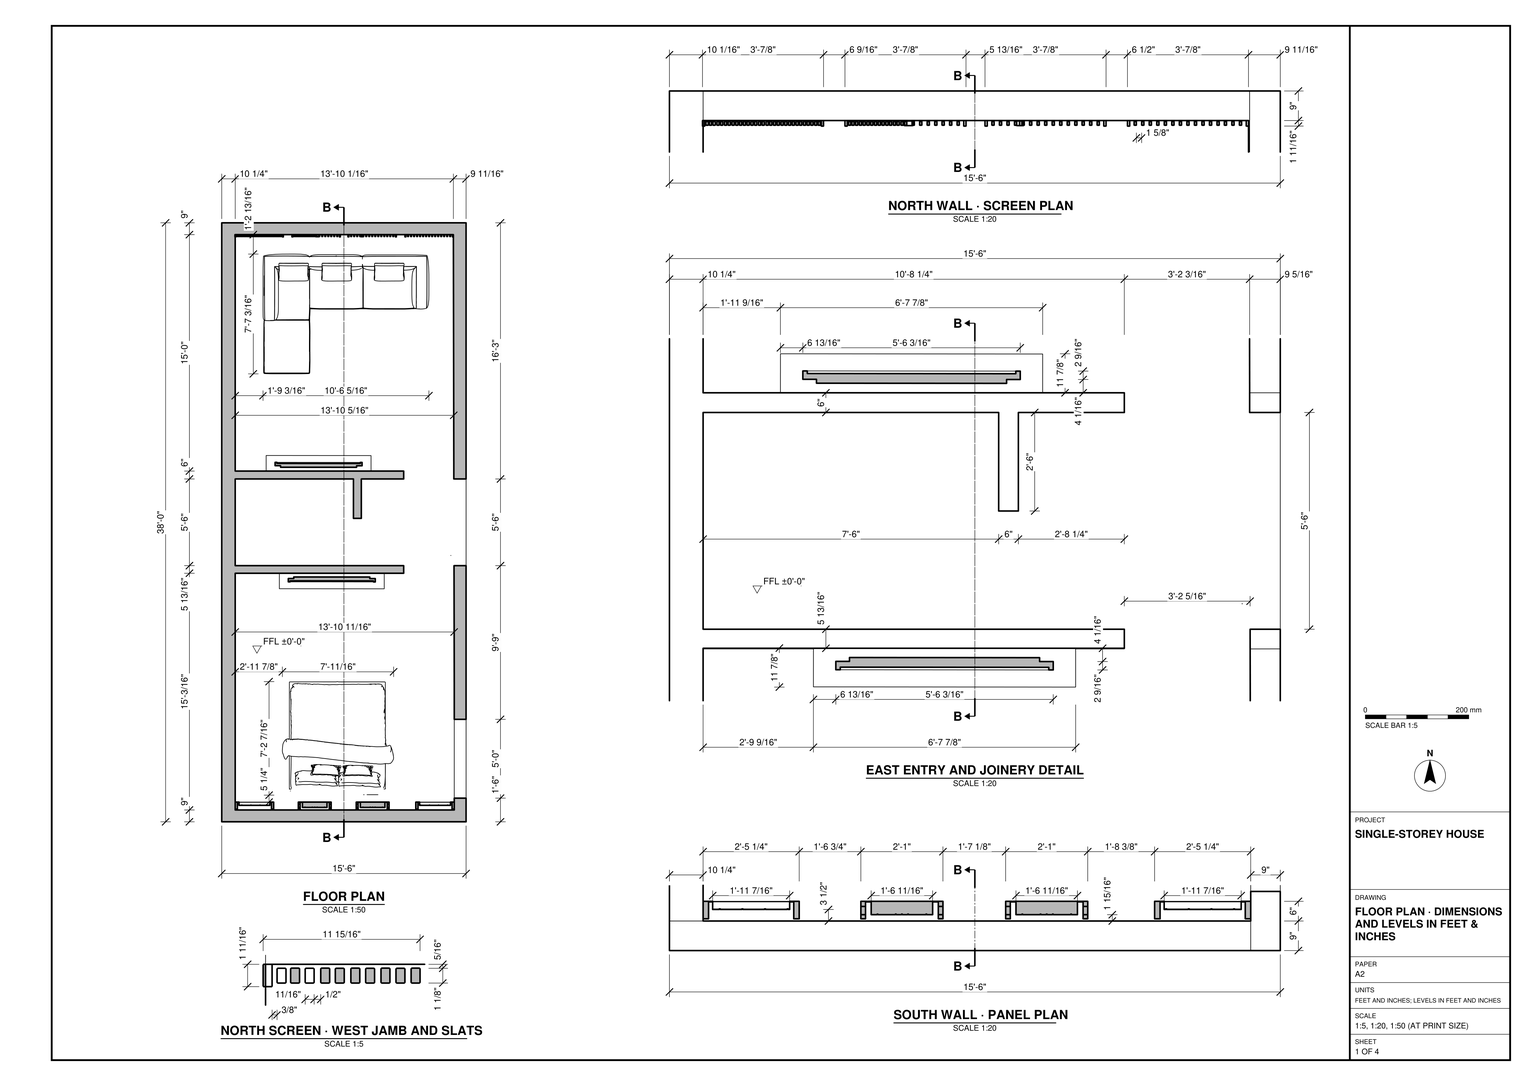
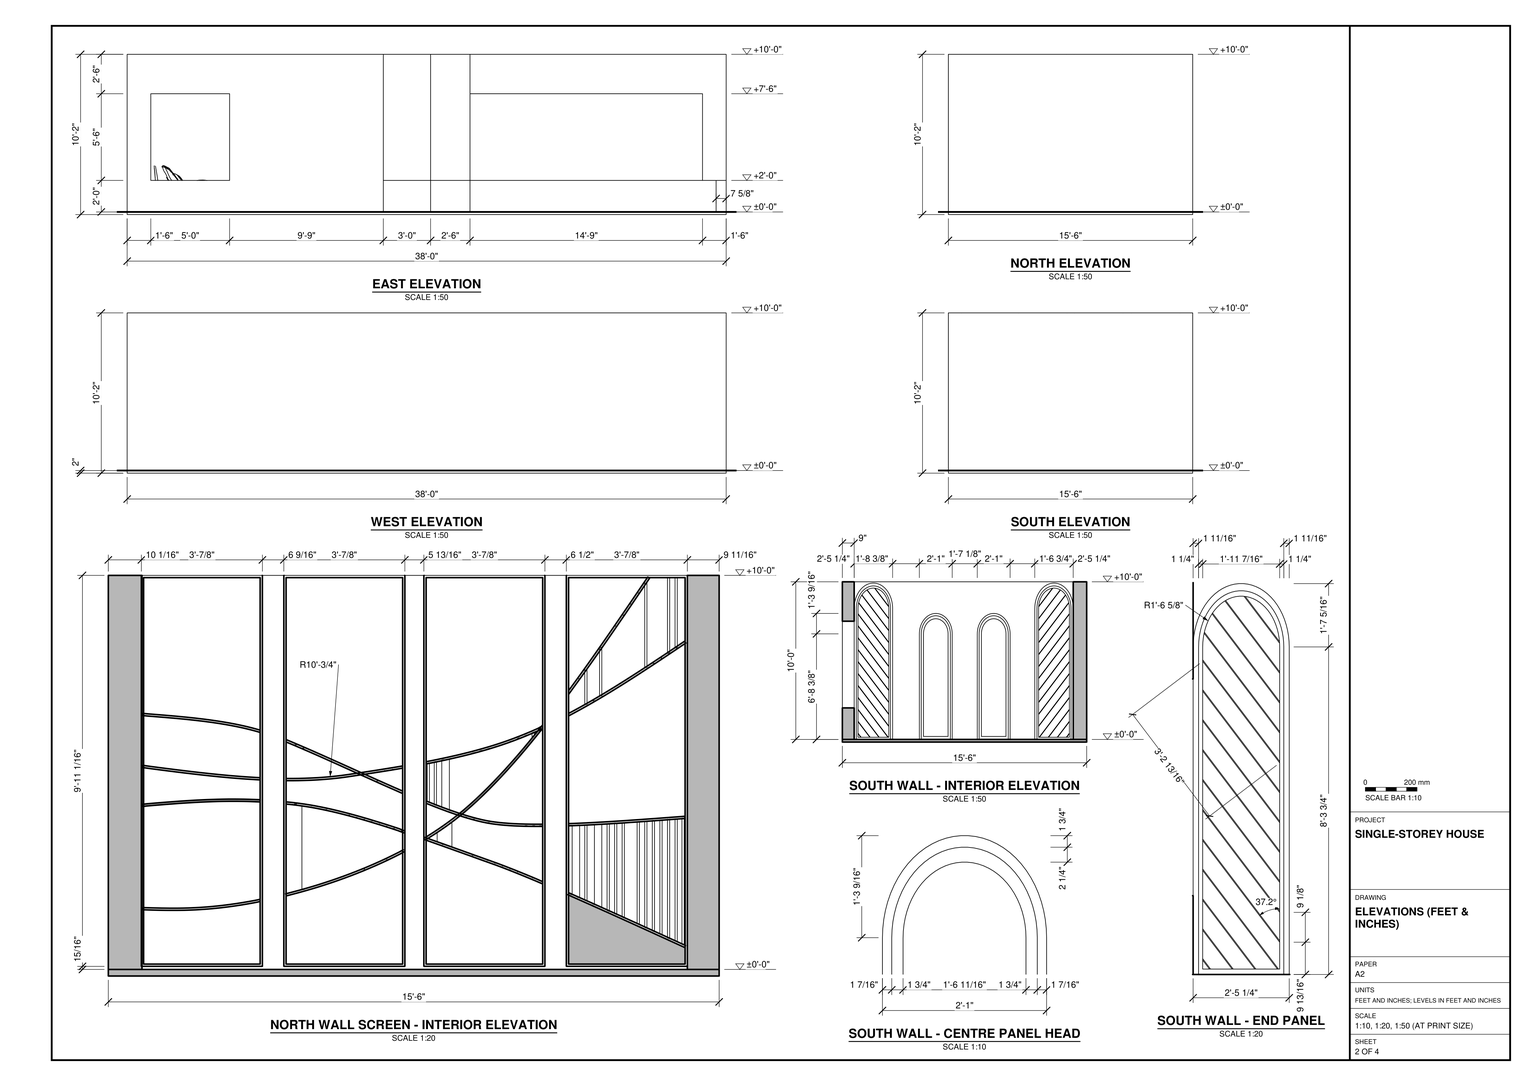
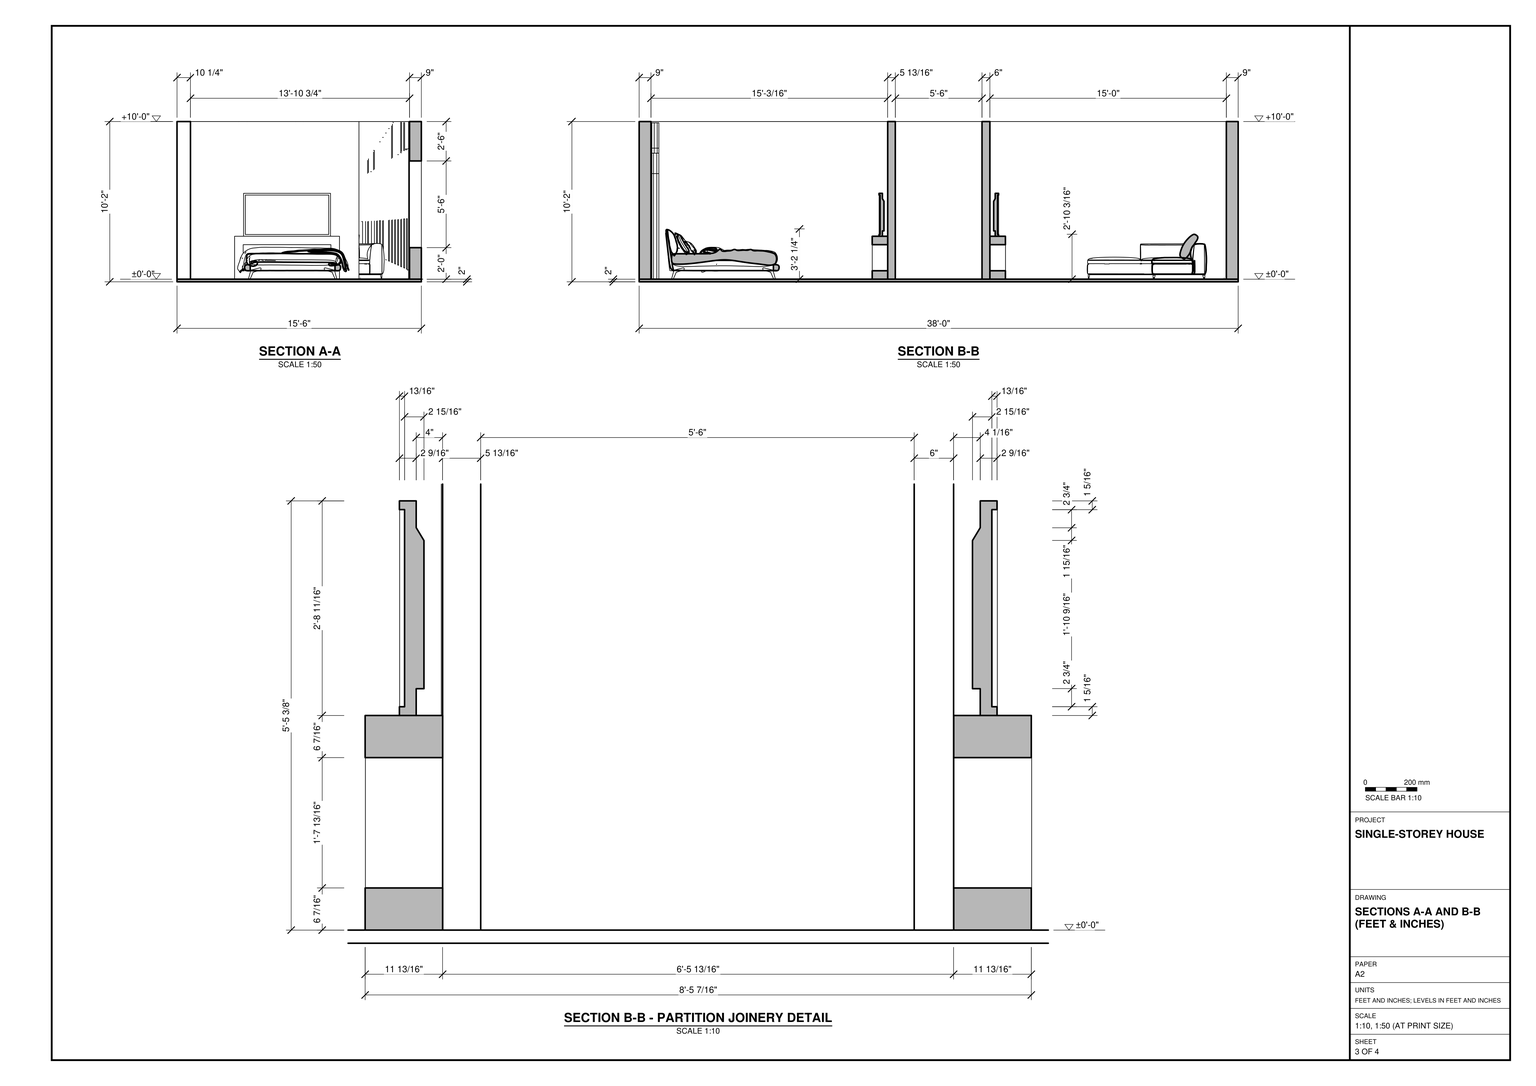
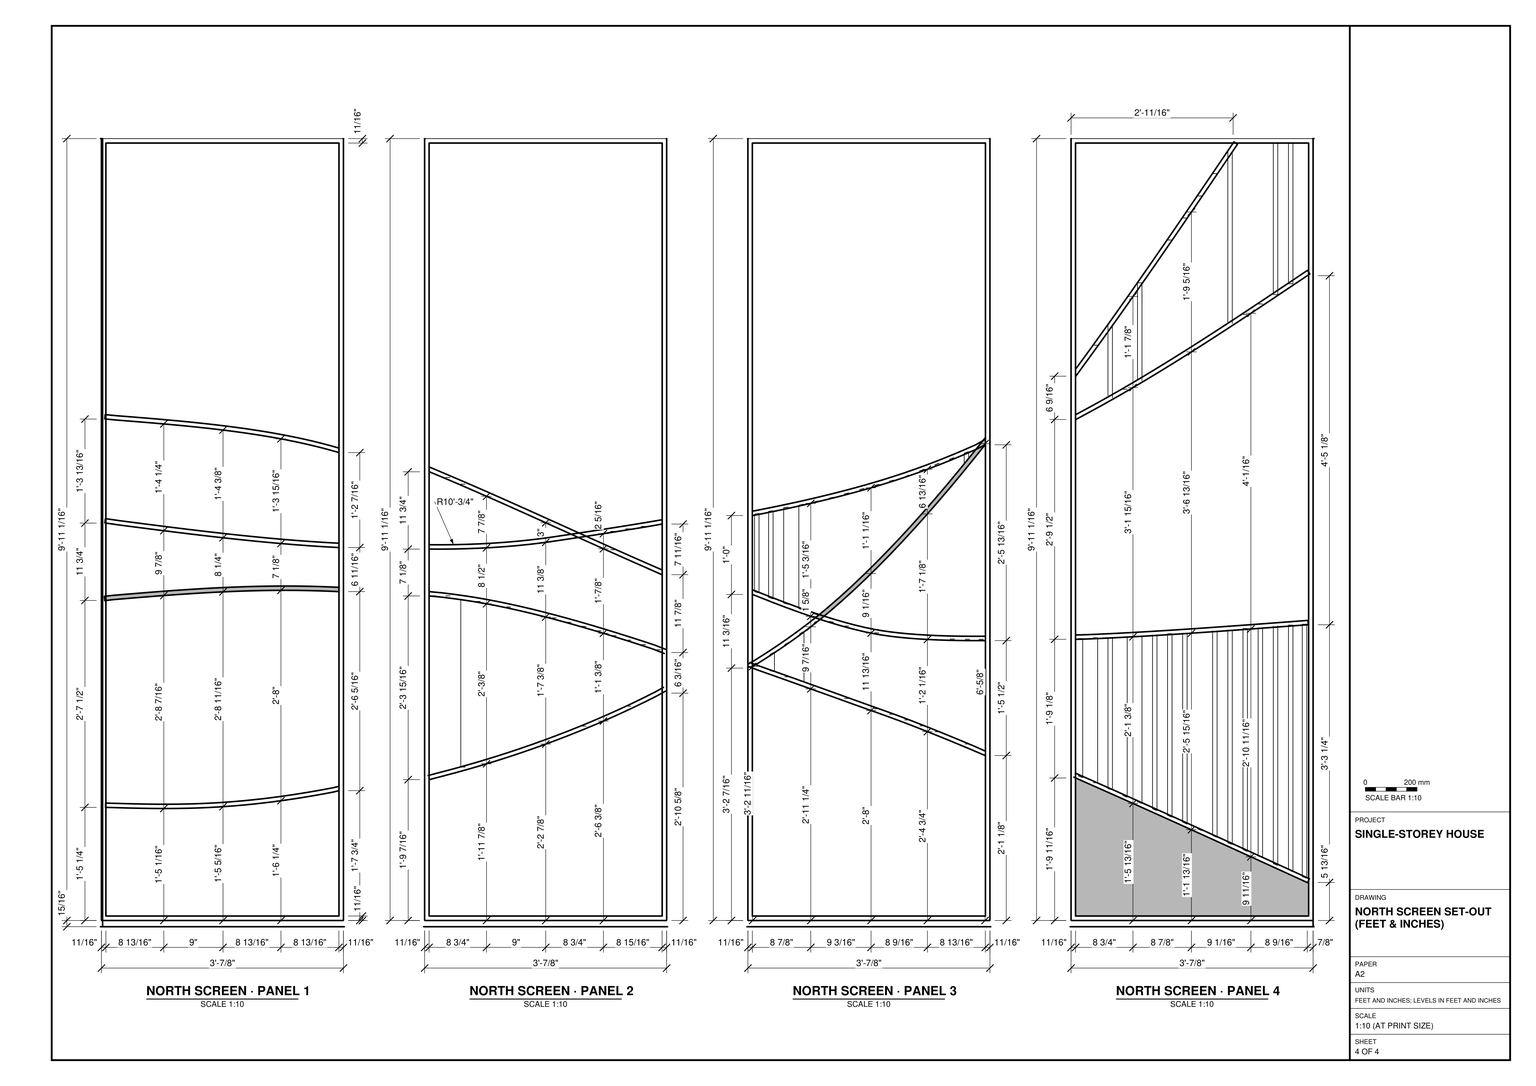
Build the house in SketchUp from task_files/diagram_01.pdf. Work in feet and inches. The rectangular footprint is 15'-6" east to west by 38'-0" north to south. Set the finished floor at ±0'-0". The overall height is 10'-2", measured from the underside of the floor slab to the wall tops.

Model the slab and perimeter walls with the thicknesses shown in plan and section. Keep the west wall continuous. Form the central entry and the two room openings in the east wall, matching their positions, sills and heads to the east elevation. Build the transverse partitions on either side of the entry, including the short return on the northern partition. Fit the low media units and their upright screens against the partition faces that look into the rooms.

Place the sectional sofa at the north end, with its chaise on the west. Behind it, model the framed screen with curved rails and vertical slats. Place the bed with its head toward the south wall and model the arched wall panels behind it, distinguishing the taller end panels from the shorter centre pair. Use the plan for furniture footprints and the interior elevations for joinery profiles. Decor and loose items may be any suitable library components. Keep shell elements and individual furniture and joinery pieces in separate groups or components, and use components for repeated parts. Save one SketchUp model as output_files/single_storey_house_with_screens_and_partition_joinery.skp.

# SketchUp Ruby script. Lengths in inches.
U = 1.inch
M = Sketchup.active_model
def pt(a) = Geom::Point3d.new(a.map { |v| v * U })
def face(e, loops, mat)
  f = e.add_face(loops[0].map { |a| pt(a) })
  loops[1..].each { |l| e.add_face(l.map { |a| pt(a) }).erase! }
  f.material = f.back_material = mat if mat
  f
end
# faces: each face lists its corners as indices into pts; further lists are holes
def faces(e, pts, list, mat = nil) = list.each { |f| face(e, (f[0].is_a?(Array) ? f : [f]).map { |l| l.map { |i| pts[i] } }, mat) }
# xy, xz, yz: faces in a plane at the given z, y or x. An outline is a flat list of corners, or four numbers for a rectangle; further outlines are holes
def ring(l) = l.size == 4 ? [[l[0], l[1]], [l[2], l[1]], [l[2], l[3]], [l[0], l[3]]] : l.each_slice(2).to_a
def flat(e, list, mat, &to3) = list.each { |f| face(e, (f[0].is_a?(Array) ? f : [f]).map { |l| ring(l).map { |u, v| to3.(u, v) } }, mat) }
def xy(e, z, list, mat = nil) = flat(e, list, mat) { |x, y| [x, y, z] }
def xz(e, y, list, mat = nil) = flat(e, list, mat) { |x, z| [x, y, z] }
def yz(e, x, list, mat = nil) = flat(e, list, mat) { |y, z| [x, y, z] }
def lines(e, pts, list) = list.each { |a, b| e.add_line(pt(pts[a]), pt(pts[b])) }
# prism: a flat outline (further loops are holes) pulled along v
def prism(e, loops, v, mat = nil)
  f = face(e, loops, mat); d = Geom::Vector3d.new(v.map { |x| x * U })
  f.pushpull(f.normal.samedirection?(d) ? d.length : -d.length)
end
def box(e, o, s, mat = nil) = prism(e, [[o, [o[0] + s[0], o[1], o[2]], [o[0] + s[0], o[1] + s[1], o[2]], [o[0], o[1] + s[1], o[2]]]], [0, 0, s[2]], mat)
def at(x, y, z, deg = 0) = Geom::Transformation.translation(pt([x, y, z])) * Geom::Transformation.rotation(ORIGIN, Z_AXIS, deg.degrees)
def axes(o, x, y, z) = Geom::Transformation.new([*x, 0, *y, 0, *z, 0, *pt(o).to_a, 1])
def part(name) = M.definitions.add(name)
# library, detail: a bought-in or finely detailed component or shape, given as its bounding box
def library(name, o, s) = part(name).tap { |d| box(d.entities, o, s) }
def detail(e, o, s) = box(e.add_group.entities, o, s)
def put(e, d, t, mat = nil) = e.add_instance(d, t).tap { |i| i.material = mat if mat }
def group(e, t, mat = nil) = e.add_group.tap { |g| g.transformation = t; g.material = mat if mat }.entities
root = M.entities
M.materials.add("Cattelan Italy Adam 3").color = [207, 207, 207]
M.materials.add("Cattelan Italy Adam 5").color = [215, 212, 206]
M.materials.add("Sumele_Dress3").color = [0, 30, 102]
M.materials.add("[Gray8]").color = [68, 68, 68]
c1 = part("Component\#1")
xy(c1.entities,0,[[0,0,138.51,0,138.51,6,10.25,6,10.25,72,100.25,72,100.25,42,106.25,42,106.25,72,138.51,72,138.51,78,10.25,78,10.25,267,0,267]])
c2 = library("Group20\#1",[157.84,-56.05,11.63],[1.18,115.45,82.67])
c3 = library("wall art",[0,0,0],[134.61,1.18,72.82])
c4 = library("Спалня Венид",[0.07,-0.07,0],[84.71,86.8,39])
c5 = part("Media cabinet")
prism(c5.entities,[[[11.8125,0,0],[11.8125,47.24,0],[11.8125,47.24,19.69],[11.8125,0,19.69]],[[11.8125,43.38,3.86],[11.8125,3.86,3.86],[11.8125,3.86,15.82],[11.8125,43.38,15.82]]],[-11.8125,0,0])
c6 = part("Framed cabinet door")
xy(c6.entities,0,[[1.18,0,3.74,39.17]],"[Gray8]")
xy(c6.entities,0.8,[[2.95,0.8,3.74,38.37]],"[Gray8]")
xy(c6.entities,2.46,[[0,2.46,1.18,36.72]])
xy(c6.entities,18.88,[[2.95,0.8,3.74,38.37]],"[Gray8]")
xy(c6.entities,19.69,[[1.18,0,3.74,39.17]],"[Gray8]")
xz(c6.entities,0,[[1.18,0,3.74,19.69]],"[Gray8]")
xz(c6.entities,0.8,[[2.95,0.8,3.74,18.88]],"[Gray8]")
xz(c6.entities,2.46,[[0,2.46,1.18,2.46,1.18,17.23,0,16.05]],"[Gray8]")
xz(c6.entities,36.72,[[0,2.46,0,16.05,1.18,17.23,1.18,2.46]],"[Gray8]")
xz(c6.entities,38.37,[[2.95,0.8,3.74,18.88]],"[Gray8]")
xz(c6.entities,39.17,[[1.18,0,3.74,19.69]],"[Gray8]")
yz(c6.entities,0,[[2.46,2.46,36.72,16.05]],"[Gray8]")
yz(c6.entities,1.18,[[[0,0,39.17,19.69],[2.46,2.46,36.72,17.23]]],"[Gray8]")
yz(c6.entities,2.95,[[0.8,0.8,38.37,18.88]])
yz(c6.entities,3.74,[[[0,0,39.17,19.69],[0.8,0.8,38.37,18.88]]],"[Gray8]")
p = [[0,2.46,16.05],[1.18,2.46,17.23],[1.18,36.72,17.23],[0,36.72,16.05]]
faces(c6.entities,p,[[0,1,2,3]],"[Gray8]")
c7 = part("LCD RACK")
put(c7.entities,c5,at(0,0,0),"[Gray8]")
put(c7.entities,c6,at(2.86,4.04,19.69))
c8 = library("Group\#4",[0,0,0],[126.29,91.17,33.41])
xy(root,0,[[0,0,177,9],[177,0,177,99,176.82,189,186,189.02,186,0],[0,9,10.25,189],[176.82,189,176.8125,195,186,195,186,189.02],[176.68,261,186,261,186,267,176.67,267],
  [176.67,267,186,456],[10.25,447,176.67,456]])
xy(root,24,[[177,18,186,78]],"Cattelan Italy Adam 3")
xy(root,90,[[177,18,186,78]],"Cattelan Italy Adam 3")
xy(root,120,[[0,0,186,0,186,195,176.8125,195,177,99,177,9,0,9],[0,9,10.25,189],[0,189,10.25,189,10.25,189.2,138.51,189.2,138.51,195,10.25,195,10.25,447,176.32,447,176.67,267,176.67,261,186,261,186,456,0,456],[100.25,231,106.25,261],[10.25,261,138.51,267]],"Cattelan Italy Adam 3")
xz(root,0,[[0,0,186,120]],"Cattelan Italy Adam 3")
xz(root,9,[[10.25,0,177,120]],"Cattelan Italy Adam 3")
xz(root,18,[[177,24,186,90]],"Cattelan Italy Adam 3")
xz(root,78,[[177,24,186,90]],"Cattelan Italy Adam 3")
xz(root,189.2,[[10.25,0,138.51,120]],"Cattelan Italy Adam 3")
xz(root,195,[[10.25,0,138.51,120],[176.8125,0,186,120]],"Cattelan Italy Adam 3")
xz(root,231,[[100.25,0,106.25,120]],"Cattelan Italy Adam 3")
xz(root,261,[[10.25,0,100.25,120],[106.25,0,138.51,120],[176.67,0,186,120]],"Cattelan Italy Adam 3")
xz(root,267,[[10.25,0,138.51,120]],"Cattelan Italy Adam 3")
xz(root,447,[[10.25,0,176.32,120]],"Cattelan Italy Adam 3")
xz(root,456,[[0,0,186,120]],"Cattelan Italy Adam 3")
yz(root,0,[[0,0,456,120]],"Cattelan Italy Adam 3")
yz(root,10.25,[[189,0,189.2,120]])
yz(root,10.25,[[9,0,189,120],[195,0,261,120],[267,0,447,120]],"Cattelan Italy Adam 3")
yz(root,100.25,[[231,0,261,120]],"Cattelan Italy Adam 3")
yz(root,106.25,[[231,0,261,120]],"Cattelan Italy Adam 3")
yz(root,138.51,[[189.2,0,195,120],[261,0,267,120]],"Cattelan Italy Adam 3")
yz(root,176.67,[[261,0,267,120]])
yz(root,177,[[[9,0,99,120],[18,24,78,90]]],"Cattelan Italy Adam 3")
yz(root,186,[[[0,0,195,120],[18,24,78,90]],[261,0,448.35,24],[448.35,0,456,24],[261,24,438,90],[438,24,456,24,456,120,261,120,261,90,438,90]],"Cattelan Italy Adam 3")
p = [[176.8125,195,0],[176.82,189,0],[177,99,0],[177,99,120],[176.8125,195,120],[176.32,447,0],
  [176.67,267,0],[176.67,267,120],[176.32,447,120],[331.54,357.28,0],[331.54,99.28,0],[174.51,202.75,0],
  [174.31,202.75,0],[186,357.28,0],[186,99,0],[313.5,99,0],[186,195,24],[186,261,24]]
faces(root,p,[[0,1,2,3,4]],"Cattelan Italy Adam 3")
faces(root,p,[[5,6,7,8]])
lines(root,p,[[9,10],[11,12],[9,13],[14,15],[16,17]])
put(root,c1,at(0,189,0))
put(root,c2,axes([95.61,218.01,-15.8],[0,1.44,0],[-1.44,0,0],[0,0,1.44]),"Cattelan Italy Adam 5")
put(root,c3,axes([177,15,0],[-1.2388,0,0],[0,-4.50921,0],[0,0,1.63454]),"Sumele_Dress3")
put(root,c4,at(130.91,106.66,0,180))
put(root,c7,axes([43.85,189.26,0],[-0.00092,-1,0],[1.69,-0.00155,0],[0,0,1.66]))
put(root,c7,axes([113.64,267,0],[0.00092,1,0],[-1.69,0.00155,0],[0,0,1.66]))
g1 = group(root,at(0,0,-2))
box(g1,[0,0,0],[186,456,2])
put(root,c8,at(31.41,341.03,0.8))
